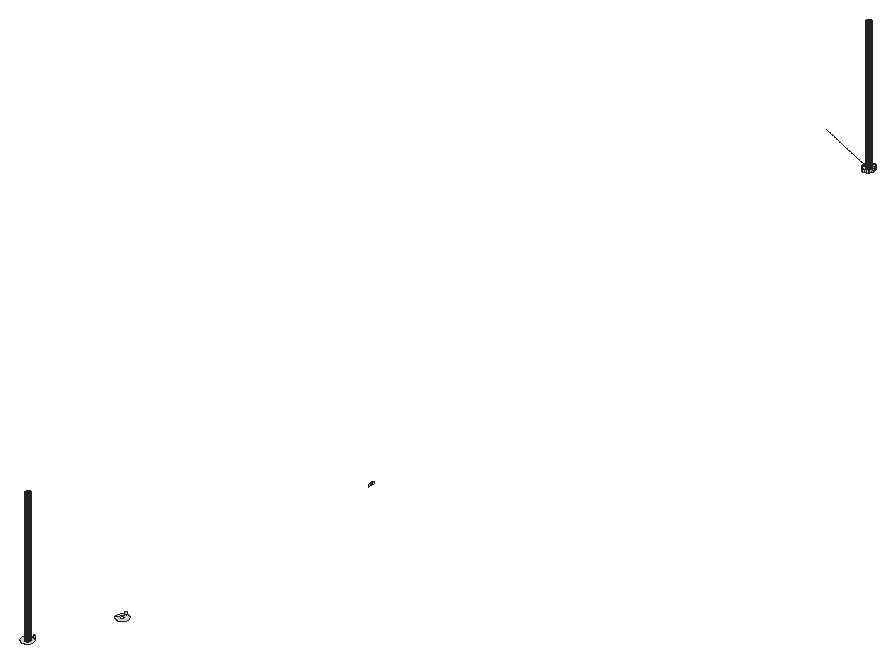
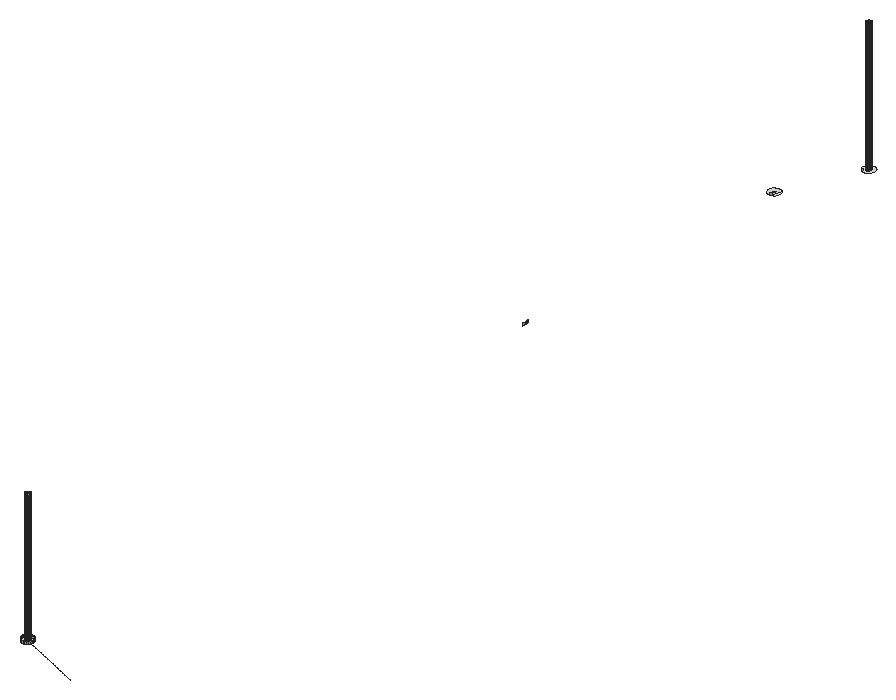
# SketchUp Ruby script. Lengths in inches.
U = 1.inch
M = Sketchup.active_model
def pt(a) = Geom::Point3d.new(a.map { |v| v * U })
def face(e, loops, mat)
  f = e.add_face(loops[0].map { |a| pt(a) })
  loops[1..].each { |l| e.add_face(l.map { |a| pt(a) }).erase! }
  f.material = f.back_material = mat if mat
  f
end
# faces: each face lists its corners as indices into pts; further lists are holes
def faces(e, pts, list, mat = nil) = list.each { |f| face(e, (f[0].is_a?(Array) ? f : [f]).map { |l| l.map { |i| pts[i] } }, mat) }
# xy, xz, yz: faces in a plane at the given z, y or x. An outline is a flat list of corners, or four numbers for a rectangle; further outlines are holes
def ring(l) = l.size == 4 ? [[l[0], l[1]], [l[2], l[1]], [l[2], l[3]], [l[0], l[3]]] : l.each_slice(2).to_a
def flat(e, list, mat, &to3) = list.each { |f| face(e, (f[0].is_a?(Array) ? f : [f]).map { |l| ring(l).map { |u, v| to3.(u, v) } }, mat) }
def xy(e, z, list, mat = nil) = flat(e, list, mat) { |x, y| [x, y, z] }
def xz(e, y, list, mat = nil) = flat(e, list, mat) { |x, z| [x, y, z] }
def yz(e, x, list, mat = nil) = flat(e, list, mat) { |y, z| [x, y, z] }
def lines(e, pts, list) = list.each { |a, b| e.add_line(pt(pts[a]), pt(pts[b])) }
# prism: a flat outline (further loops are holes) pulled along v
def prism(e, loops, v, mat = nil)
  f = face(e, loops, mat); d = Geom::Vector3d.new(v.map { |x| x * U })
  f.pushpull(f.normal.samedirection?(d) ? d.length : -d.length)
end
def box(e, o, s, mat = nil) = prism(e, [[o, [o[0] + s[0], o[1], o[2]], [o[0] + s[0], o[1] + s[1], o[2]], [o[0], o[1] + s[1], o[2]]]], [0, 0, s[2]], mat)
def at(x, y, z, deg = 0) = Geom::Transformation.translation(pt([x, y, z])) * Geom::Transformation.rotation(ORIGIN, Z_AXIS, deg.degrees)
def axes(o, x, y, z) = Geom::Transformation.new([*x, 0, *y, 0, *z, 0, *pt(o).to_a, 1])
def part(name) = M.definitions.add(name)
# library, detail: a bought-in or finely detailed component or shape, given as its bounding box
def library(name, o, s) = part(name).tap { |d| box(d.entities, o, s) }
def detail(e, o, s) = box(e.add_group.entities, o, s)
def put(e, d, t, mat = nil) = e.add_instance(d, t).tap { |i| i.material = mat if mat }
def group(e, t, mat = nil) = e.add_group.tap { |g| g.transformation = t; g.material = mat if mat }.entities
root = M.entities
M.materials.add("[Color_000]").color = [255, 255, 255]
xy(root,321.27,[[[945.45,768.58,945.85,768.67,946.22,768.85,946.53,769.125,946.75,769.47,946.88,769.86,946.91,770.27,946.82,770.67,946.64,771.04,946.37,771.34,946.02,771.57,945.88,771.62,945.63,771.7,945.22,771.73,944.82,771.64,944.45,771.46,944.14,771.19,943.92,770.84,943.79,770.45,943.76,770.04,943.85,769.64,944.03,769.27,944.3,768.96,944.63,768.75,944.65,768.74,945.04,768.61],[945.38,769.53,945.22,769.54,945.06,769.59,945.01,769.62,944.92,769.68,944.8125,769.8,944.74,769.95,944.71,770.11,944.72,770.27,944.77,770.43,944.86,770.57,944.98,770.68,945.13,770.75,945.29,770.78,945.45,770.77,945.51,770.76,945.61,770.72,945.75,770.63,945.86,770.51,945.93,770.36,945.96,770.2,945.95,770.04,945.9,769.88,945.8125,769.74,945.6875,769.63,945.54,769.56]],[945.01,769.62,945.51,770.76,945.45,770.77,945.29,770.78,945.13,770.75,944.98,770.68,944.86,770.57,944.77,770.43,944.72,770.27,944.71,770.11,944.74,769.95,944.8125,769.8,944.92,769.68],[[955.0625,788.75,955.46,788.84,955.83,789.02,956.14,789.29,956.37,789.64,956.49,790.03,956.52,790.4375,956.4375,790.84,956.25,791.21,955.98,791.51,955.64,791.74,955.25,791.87,954.84,791.89,954.7,791.87,953.64,789.44,953.92,789.13,954.26,788.91,954.65,788.78],[954.83,789.7,954.67,789.76,954.54,789.85,954.43,789.97,954.35,790.12,954.32,790.28,954.33,790.44,954.38,790.6,954.47,790.74,954.6,790.84,954.74,790.92,954.9,790.95,955.07,790.94,955.22,790.89,955.36,790.8,955.47,790.68,955.54,790.53,955.58,790.37,955.57,790.2,955.52,790.05,955.42,789.91,955.3,789.8,955.15,789.73,954.99,789.7]],[953.64,789.44,954.7,791.87,954.43,791.8125,954.07,791.63,953.76,791.35,953.53,791.01,953.4,790.62,953.38,790.21,953.46,789.81],[957.4375,1039.9,957.03,1039.93,956.64,1040.06,956.29,1040.28,956.02,1040.59,955.84,1040.96,955.75,1041.36,955.78,1041.77,955.89,1042.1,956.75,1041.72,956.71,1041.59,956.7,1041.43,956.73,1041.27,956.8,1041.12,956.91,1041,957.05,1040.91,957.21,1040.85,957.37,1040.84,957.53,1040.88,957.68,1040.95,957.8,1041.0625,957.89,1041.2,957.9,1041.22,958.76,1040.85,958.74,1040.79,958.51,1040.44,958.21,1040.17,957.84,1039.98],
  [[957.4375,1039.9,957.84,1039.98,958.21,1040.17,958.51,1040.44,958.74,1040.79,958.87,1041.18,958.9,1041.59,958.8125,1041.99,958.63,1042.36,958.36,1042.66,958.01,1042.89,957.62,1043.02,957.21,1043.04,956.81,1042.96,956.44,1042.78,956.13,1042.5,955.91,1042.16,955.78,1041.77,955.75,1041.36,955.84,1040.96,956.02,1040.59,956.29,1040.28,956.64,1040.06,957.03,1039.93],[957.37,1040.84,957.21,1040.85,957.05,1040.91,956.91,1041,956.8,1041.12,956.73,1041.27,956.7,1041.43,956.71,1041.59,956.75,1041.72,956.76,1041.75,956.85,1041.89,956.97,1041.99,957.12,1042.07,957.28,1042.1,957.44,1042.09,957.6,1042.04,957.74,1041.95,957.85,1041.83,957.92,1041.68,957.95,1041.52,957.94,1041.35,957.9,1041.22,957.89,1041.2,957.8,1041.0625,957.68,1040.95,957.53,1040.88]]])
xy(root,321.27,[[945.38,769.53,945.54,769.56,945.6875,769.63,945.8125,769.74,945.9,769.88,945.95,770.04,945.96,770.2,945.93,770.36,945.86,770.51,945.75,770.63,945.61,770.72,945.51,770.76,945.01,769.62,945.06,769.59,945.22,769.54],[957.37,1040.84,957.21,1040.85,957.05,1040.91,956.91,1041,956.8,1041.12,956.73,1041.27,956.7,1041.43,956.71,1041.59,956.75,1041.72,957.9,1041.22,957.89,1041.2,957.8,1041.0625,957.68,1040.95,957.53,1040.88],[957.9,1041.22,956.75,1041.72,956.76,1041.75,956.85,1041.89,956.97,1041.99,957.12,1042.07,957.28,1042.1,957.44,1042.09,957.6,1042.04,957.74,1041.95,957.85,1041.83,957.92,1041.68,957.95,1041.52,957.94,1041.35]],"[Color_000]")
p = [[945.06,769.59,321.27],[945.22,769.54,321.27],[945.22,769.54,357.27],[945.06,769.59,357.27],[945.38,769.53,321.27],[945.38,769.53,357.27],
  [945.54,769.56,321.27],[945.54,769.56,357.27],[944.92,769.68,321.27],[945.01,769.62,321.27],[944.92,769.68,357.27],[945.6875,769.63,321.27],
  [945.6875,769.63,357.27],[945.8125,769.74,321.27],[945.8125,769.74,357.27],[944.8125,769.8,321.27],[944.8125,769.8,357.27],[945.9,769.88,321.27],
  [945.9,769.88,357.27],[944.74,769.95,321.27],[944.74,769.95,357.27],[945.95,770.04,321.27],[945.95,770.04,357.27],[945.96,770.2,321.27],
  [945.96,770.2,357.27],[945.93,770.36,321.27],[945.93,770.36,357.27],[944.86,770.57,321.27],[944.77,770.43,321.27],[944.77,770.43,357.27],
  [944.86,770.57,357.27],[945.86,770.51,321.27],[945.86,770.51,357.27],[945.75,770.63,321.27],[945.75,770.63,357.27],[944.98,770.68,321.27],
  [944.98,770.68,357.27],[945.13,770.75,321.27],[945.13,770.75,357.27],[945.29,770.78,321.27],[945.29,770.78,357.27],[945.61,770.72,321.27],
  [945.51,770.76,321.27],[945.45,770.77,321.27],[945.45,770.77,357.27],[945.61,770.72,357.27],[946.02,771.57,321.27],[945.88,771.62,321.27],
  [945.63,771.7,321.27],[945.63,771.7,321.86],[946.02,771.57,321.86],[954.84,791.89,321.27],[954.7,791.87,321.27],[954.43,791.8125,321.27],
  [954.43,791.8125,321.86],[954.84,791.89,321.86],[960.32,867.76,321.27],[960.5,867.4,321.27],[960.5,867.4,321.86],[960.32,867.76,321.86],
  [960.23,868.17,321.27],[960.23,868.17,321.86],[960.26,868.58,321.27],[960.26,868.58,321.86],[960.39,868.97,321.27],[960.39,868.97,321.86],
  [956.64,1040.06,321.27],[957.03,1039.93,321.27],[957.03,1039.93,321.86],[956.64,1040.06,321.86],[957.4375,1039.9,321.27],[957.4375,1039.9,321.86],
  [957.84,1039.98,321.27],[957.84,1039.98,321.86],[958.21,1040.17,321.27],[958.21,1040.17,321.86],[956.29,1040.28,321.27],[956.29,1040.28,321.86],
  [958.51,1040.44,321.27],[958.51,1040.44,321.86],[956.02,1040.59,321.27],[956.02,1040.59,321.86],[958.74,1040.79,321.27],[958.74,1040.79,321.86],
  [955.84,1040.96,321.27],[955.84,1040.96,321.86],[957.21,1040.85,321.27],[957.37,1040.84,321.27],[957.37,1040.84,357.27],[957.21,1040.85,357.27],
  [957.53,1040.88,321.27],[957.53,1040.88,357.27],[958.76,1040.85,321.27],[958.87,1041.18,321.27],[958.87,1041.18,321.86],[956.91,1041,321.27],
  [957.05,1040.91,321.27],[957.05,1040.91,357.27],[956.91,1041,357.27],[957.68,1040.95,321.27],[957.68,1040.95,357.27],[955.75,1041.36,321.27],
  [955.75,1041.36,321.86],[956.8,1041.12,321.27],[956.8,1041.12,357.27],[957.8,1041.0625,321.27],[957.8,1041.0625,357.27],[956.73,1041.27,321.27],
  [956.73,1041.27,357.27],[957.89,1041.2,321.27],[957.89,1041.2,357.27],[957.9,1041.22,321.27],[957.94,1041.35,321.27],[957.94,1041.35,357.27],
  [958.9,1041.59,321.27],[958.9,1041.59,321.86],[956.7,1041.43,321.27],[956.7,1041.43,357.27],[955.78,1041.77,321.27],[955.78,1041.77,321.86],
  [956.71,1041.59,321.27],[956.71,1041.59,357.27],[957.95,1041.52,321.27],[957.95,1041.52,357.27],[957.92,1041.68,321.27],[957.92,1041.68,357.27],
  [956.76,1041.75,321.27],[956.75,1041.72,321.27],[956.76,1041.75,357.27],[958.8125,1041.99,321.27],[958.8125,1041.99,321.86],[956.85,1041.89,321.27],
  [956.85,1041.89,357.27],[957.85,1041.83,321.27],[957.85,1041.83,357.27],[955.91,1042.16,321.27],[955.89,1042.1,321.27],[955.91,1042.16,321.86],
  [957.74,1041.95,321.27],[957.74,1041.95,357.27],[956.97,1041.99,321.27],[956.97,1041.99,357.27],[957.6,1042.04,321.27],[957.6,1042.04,357.27],
  [957.12,1042.07,321.27],[957.12,1042.07,357.27],[957.44,1042.09,321.27],[957.44,1042.09,357.27],[958.63,1042.36,321.27],[958.63,1042.36,321.86],
  [957.28,1042.1,321.27],[957.28,1042.1,357.27],[956.13,1042.5,321.27],[956.13,1042.5,321.86],[958.36,1042.66,321.27],[958.36,1042.66,321.86],
  [956.44,1042.78,321.27],[956.44,1042.78,321.86],[958.01,1042.89,321.27],[958.01,1042.89,321.86],[956.81,1042.96,321.27],[956.81,1042.96,321.86],
  [957.62,1043.02,321.27],[957.62,1043.02,321.86],[957.21,1043.04,321.27],[957.21,1043.04,321.86],[939.38,1049.29,321.27]]
faces(root,p,[[0,1,2,3],[1,4,5,2],[4,6,7,5],[8,9,0,3,10],[6,11,12,7],[11,13,14,12],[15,8,10,16],[13,17,18,14],
  [19,15,16,20],[17,21,22,18],[21,23,24,22],[23,25,26,24],[27,28,29,30],[25,31,32,26],[31,33,34,32],[35,27,30,36],
  [37,35,36,38],[39,37,38,40],[41,42,43,44,45],[43,39,40,44],[86,87,88,89],[87,90,91,88],[95,96,97,98],[96,86,89,97],
  [90,99,100,91],[103,95,98,104],[99,105,106,100],[107,103,104,108],[105,109,110,106],[109,111,112,113,110],[116,107,108,117],[120,116,117,121],
  [112,122,123,113],[122,124,125,123],[126,127,120,121,128],[131,126,128,132],[124,133,134,125],[133,138,139,134],[140,131,132,141],[138,142,143,139],
  [144,140,141,145],[142,146,147,143],[150,144,145,151],[146,150,151,147]],"[Color_000]")
faces(root,p,[[46,47,48,49,50],[51,52,53,54,55],[56,57,58,59],[60,56,59,61],[62,60,61,63],[64,62,63,65],[66,67,68,69],[67,70,71,68],
  [70,72,73,71],[72,74,75,73],[76,66,69,77],[74,78,79,75],[80,76,77,81],[78,82,83,79],[84,80,81,85],[82,92,93,94,83],
  [101,84,85,102],[93,114,115,94],[118,101,102,119],[114,129,130,115],[135,136,118,119,137],[129,148,149,130],[152,135,137,153],[148,154,155,149],
  [156,152,153,157],[154,158,159,155],[160,156,157,161],[158,162,163,159],[164,160,161,165],[162,164,165,163]])
lines(root,p,[[136,166]])
